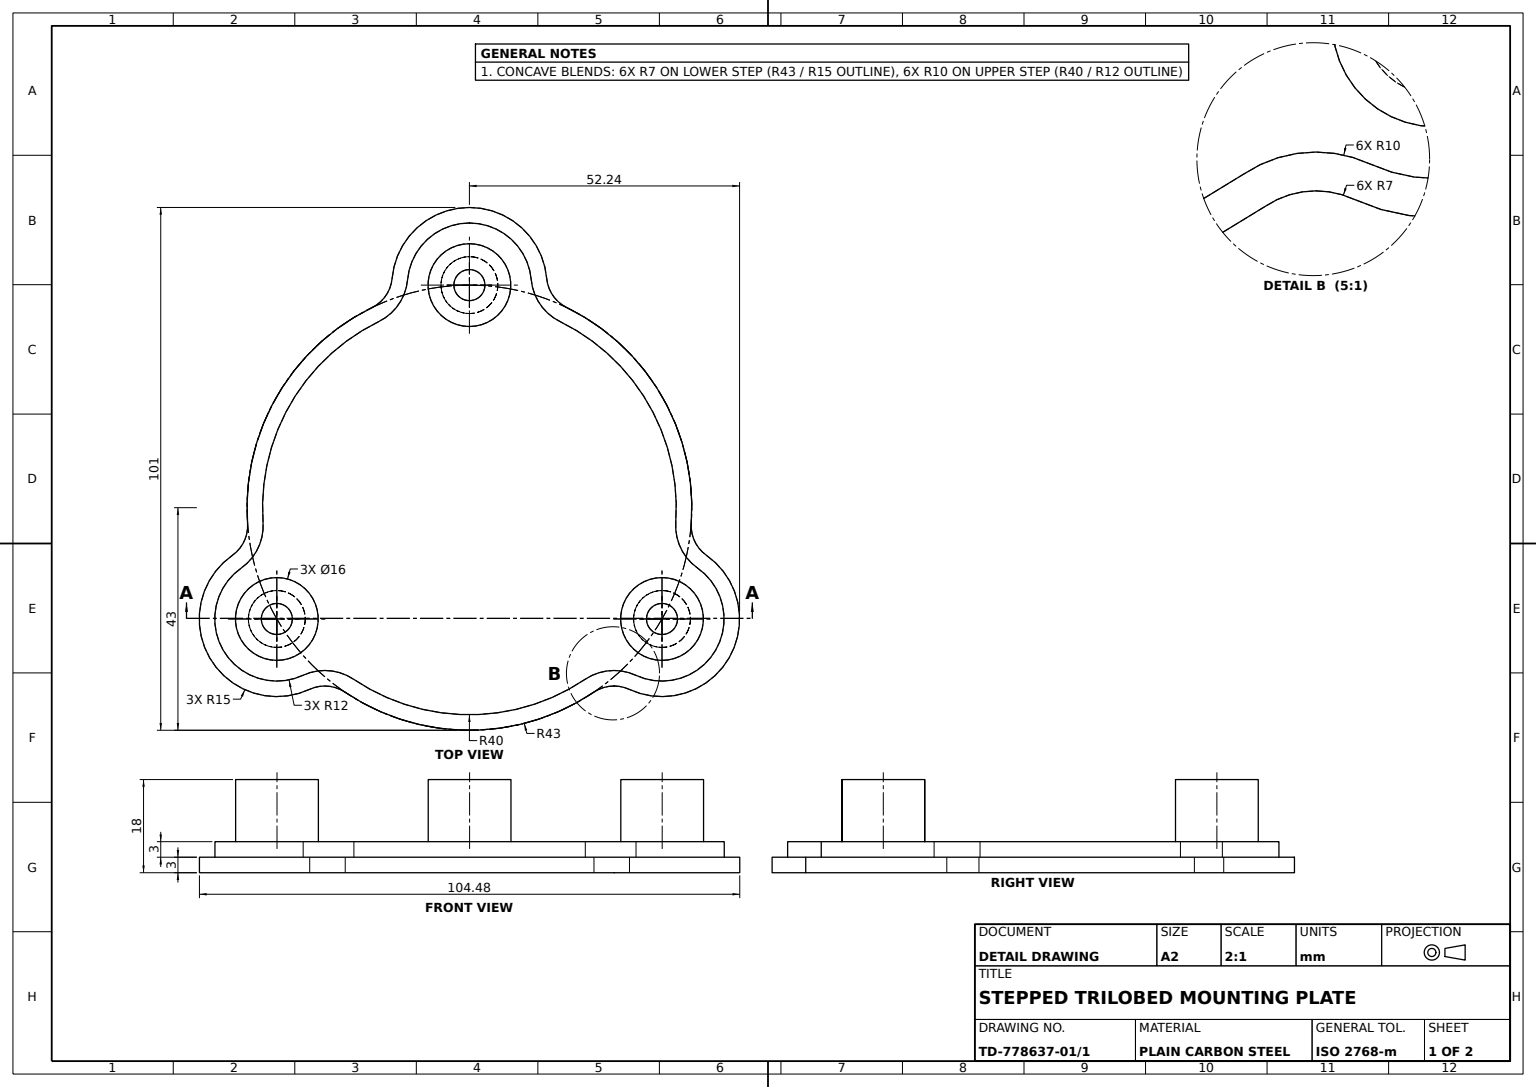
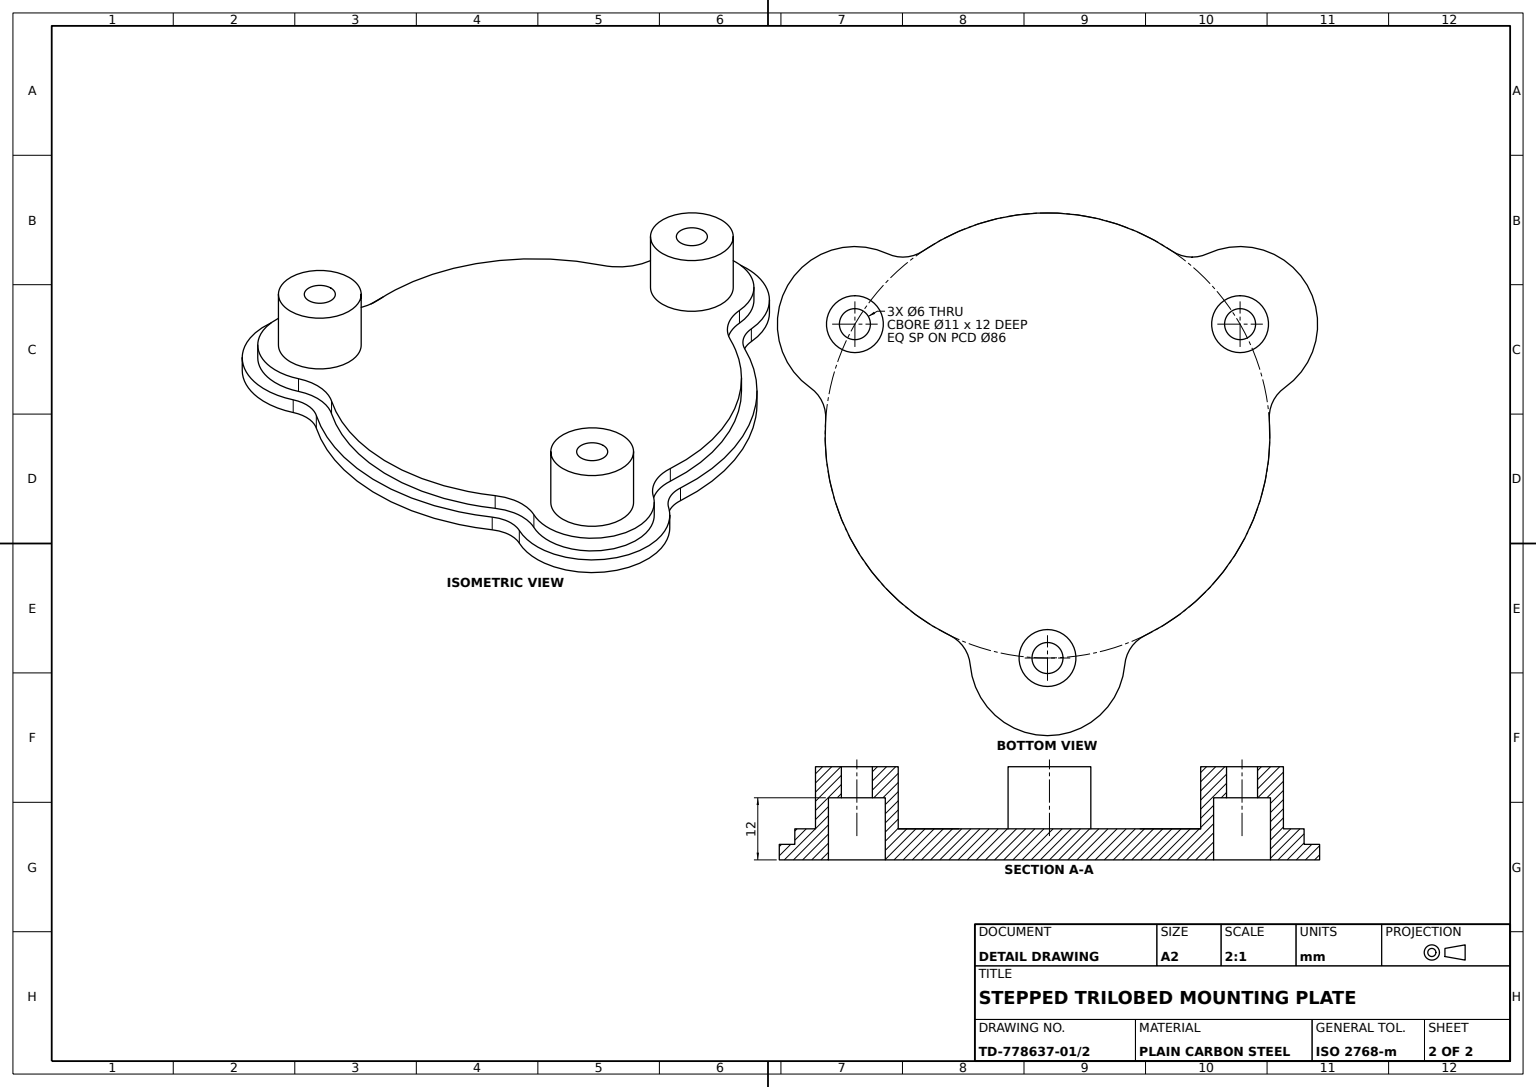
solid
v1 (27.963727,3,34.449125)
v2 (30.91498,3,35.101676)
e1 v1 v2 CIRCLE(AX(P(27.963727,3,41.449125),D(0,-1,0),D(0,0,1)),7)
v3 (27.963727,0,34.449125)
e2 v1 v3 LINE
v4 (30.91498,0,35.101676)
e3 v3 v4 CIRCLE(AX(P(27.963727,0,41.449125),D(0,-1,0),D(0,0,1)),7)
e4 v2 v4 LINE
face CYL(AX(P(27.963727,3,41.449125),D(0,-1,0),D(0,0,-1)),7) rev [-e1 e2 e3 -e4]
v5 (-37.239092,12,27)
v6 (-37.239092,12,16)
e5 v5 v6 CIRCLE(AX(P(-37.239092,12,21.5),D(0,-1,0),D(0,0,-1)),5.5)
v7 (-37.239092,0,27)
e6 v5 v7 LINE
v8 (-37.239092,0,16)
e7 v7 v8 CIRCLE(AX(P(-37.239092,0,21.5),D(0,-1,0),D(0,0,-1)),5.5)
e8 v6 v8 LINE
face CYL(AX(P(-37.239092,12,21.5),D(0,-1,0),D(0,0,-1)),5.5) rev [-e5 e6 e7 -e8]
v9 (-37.239092,18,18.5)
v10 (-37.239092,12,18.5)
e9 v9 v10 LINE
v11 (-37.239092,12,24.5)
e10 v10 v11 CIRCLE(AX(P(-37.239092,12,21.5),D(0,-1,0),D(0,0,-1)),3)
v12 (-37.239092,18,24.5)
e11 v12 v11 LINE
e12 v12 v9 CIRCLE(AX(P(-37.239092,18,21.5),D(0,1,0),D(0,0,1)),3)
face CYL(AX(P(-37.239092,22,21.5),D(0,-1,0),D(0,0,-1)),3) rev [e9 e10 -e11 e12]
v13 (-17.531306,3,-35.953488)
v14 (-39.902287,3,2.794188)
e13 v13 v14 CIRCLE(AX(P(0,3,0),D(0,1,0),D(0,0,1)),40)
v15 (-39.902287,6,2.794188)
e14 v15 v14 LINE
v16 (-17.531306,6,-35.953488)
e15 v16 v15 CIRCLE(AX(P(0,6,0),D(0,1,0),D(0,0,1)),40)
e16 v16 v13 LINE
face CYL(AX(P(0,6,0),D(0,-1,0),D(0,0,-1)),40) [e13 -e14 -e15 e16]
v17 (-44.132965,6,11.677856)
v18 (-44.132965,3,11.677856)
e17 v17 v18 LINE
v19 (-32.179802,3,32.381341)
e18 v18 v19 CIRCLE(AX(P(-37.239092,3,21.5),D(0,1,0),D(0,0,1)),12)
v20 (-32.179802,6,32.381341)
e19 v20 v19 LINE
e20 v17 v20 CIRCLE(AX(P(-37.239092,6,21.5),D(0,1,0),D(0,0,1)),12)
face CYL(AX(P(-37.239092,6,21.5),D(0,-1,0),D(0,0,-1)),12) [e17 e18 -e19 -e20]
v21 (-30.91498,0,35.101676)
v22 (-27.963727,0,34.449125)
e21 v21 v22 CIRCLE(AX(P(-27.963727,0,41.449125),D(0,-1,0),D(0,0,-1)),7)
v23 (-27.963727,3,34.449125)
e22 v23 v22 LINE
v24 (-30.91498,3,35.101676)
e23 v24 v23 CIRCLE(AX(P(-27.963727,3,41.449125),D(0,-1,0),D(0,0,-1)),7)
e24 v24 v21 LINE
face CYL(AX(P(-27.963727,3,41.449125),D(0,-1,0),D(0,0,-1)),7) rev [e21 -e22 -e23 e24]
v25 (-37.239092,6,29.5)
v26 (-37.239092,18,29.5)
e25 v25 v26 LINE
v27 (-37.239092,18,13.5)
e26 v27 v26 CIRCLE(AX(P(-37.239092,18,21.5),D(0,1,0),D(0,0,1)),8)
v28 (-37.239092,6,13.5)
e27 v28 v27 LINE
e28 v28 v25 CIRCLE(AX(P(-37.239092,6,21.5),D(0,1,0),D(0,0,1)),8)
face CYL(AX(P(-37.239092,0,21.5),D(0,1,0),D(0,0,1)),8) [e25 -e26 -e27 e28]
v29 (-27.963727,3,31.449125)
e29 v19 v29 CIRCLE(AX(P(-27.963727,3,41.449125),D(0,-1,0),D(0,0,1)),10)
v30 (-27.963727,6,31.449125)
e30 v30 v29 LINE
e31 v20 v30 CIRCLE(AX(P(-27.963727,6,41.449125),D(0,-1,0),D(0,0,1)),10)
face CYL(AX(P(-27.963727,6,41.449125),D(0,-1,0),D(0,0,-1)),10) rev [e19 e29 -e30 -e31]
e32 v26 v27 CIRCLE(AX(P(-37.239092,18,21.5),D(0,1,0),D(0,0,1)),8)
e33 v9 v12 CIRCLE(AX(P(-37.239092,18,21.5),D(0,1,0),D(0,0,1)),3)
face PLANE(AX(P(-37.239092,18,21.5),D(0,1,0),D(0,0,1))) [e26 e32] [-e33 -e12]
e34 v25 v28 CIRCLE(AX(P(-37.239092,6,21.5),D(0,1,0),D(0,0,1)),8)
face CYL(AX(P(-37.239092,0,21.5),D(0,1,0),D(0,0,1)),8) [-e32 -e25 e34 e27]
v31 (14.941454,3,-44.323996)
v32 (14.941454,0,-44.323996)
e35 v31 v32 LINE
v33 (0,0,-58)
e36 v32 v33 CIRCLE(AX(P(0,0,-43),D(0,1,0),D(0,0,1)),15)
v34 (0,3,-58)
e37 v34 v33 LINE
e38 v31 v34 CIRCLE(AX(P(0,3,-43),D(0,1,0),D(0,0,1)),15)
face CYL(AX(P(0,3,-43),D(0,-1,0),D(0,0,-1)),15) [e35 e36 -e37 -e38]
v35 (37.239092,18,18.5)
v36 (37.239092,18,24.5)
e39 v35 v36 CIRCLE(AX(P(37.239092,18,21.5),D(0,1,0),D(0,0,1)),3)
e40 v36 v35 CIRCLE(AX(P(37.239092,18,21.5),D(0,1,0),D(0,0,1)),3)
v37 (37.239092,18,13.5)
v38 (37.239092,18,29.5)
e41 v37 v38 CIRCLE(AX(P(37.239092,18,21.5),D(0,1,0),D(0,0,1)),8)
e42 v38 v37 CIRCLE(AX(P(37.239092,18,21.5),D(0,1,0),D(0,0,1)),8)
face PLANE(AX(P(37.239092,18,21.5),D(0,1,0),D(0,0,1))) [-e39 -e40] [e41 e42]
v39 (18.846153,3,-38.65)
v40 (18.846153,0,-38.65)
e43 v39 v40 LINE
e44 v40 v32 CIRCLE(AX(P(21.914132,0,-44.94186),D(0,-1,0),D(0,0,1)),7)
e45 v39 v31 CIRCLE(AX(P(21.914132,3,-44.94186),D(0,-1,0),D(0,0,1)),7)
face CYL(AX(P(21.914132,3,-44.94186),D(0,-1,0),D(0,0,-1)),7) rev [e43 e44 -e35 -e45]
v41 (24.048805,3,35.646248)
v42 (24.048805,0,35.646248)
e46 v41 v42 LINE
v43 (-24.048805,3,35.646248)
e47 v43 v41 CIRCLE(AX(P(0,3,0),D(0,1,0),D(0,0,1)),43)
v44 (-24.048805,0,35.646248)
e48 v43 v44 LINE
e49 v44 v42 CIRCLE(AX(P(0,0,0),D(0,1,0),D(0,0,1)),43)
face CYL(AX(P(0,3,0),D(0,-1,0),D(0,0,-1)),43) [-e46 -e47 e48 e49]
v45 (27.963727,6,31.449125)
v46 (27.963727,3,31.449125)
e50 v45 v46 LINE
v47 (32.179802,3,32.381341)
e51 v46 v47 CIRCLE(AX(P(27.963727,3,41.449125),D(0,-1,0),D(0,0,1)),10)
v48 (32.179802,6,32.381341)
e52 v48 v47 LINE
e53 v45 v48 CIRCLE(AX(P(27.963727,6,41.449125),D(0,-1,0),D(0,0,1)),10)
face CYL(AX(P(27.963727,6,41.449125),D(0,-1,0),D(0,0,-1)),10) rev [e50 e51 -e52 -e53]
v49 (37.239092,12,16)
v50 (37.239092,0,16)
e54 v49 v50 LINE
v51 (37.239092,12,27)
e55 v51 v49 CIRCLE(AX(P(37.239092,12,21.5),D(0,-1,0),D(0,0,-1)),5.5)
v52 (37.239092,0,27)
e56 v51 v52 LINE
e57 v52 v50 CIRCLE(AX(P(37.239092,0,21.5),D(0,-1,0),D(0,0,-1)),5.5)
face CYL(AX(P(37.239092,12,21.5),D(0,-1,0),D(0,0,-1)),5.5) rev [-e54 -e55 e56 e57]
v53 (45.856433,3,9.22232)
v54 (45.856433,0,9.22232)
e58 v53 v54 LINE
v55 (42.894959,0,3.003752)
e59 v54 v55 CIRCLE(AX(P(49.877859,0,3.492735),D(0,-1,0),D(0,0,-1)),7)
v56 (42.894959,3,3.003752)
e60 v56 v55 LINE
e61 v53 v56 CIRCLE(AX(P(49.877859,3,3.492735),D(0,-1,0),D(0,0,-1)),7)
face CYL(AX(P(49.877859,3,3.492735),D(0,-1,0),D(0,0,-1)),7) rev [e58 e59 -e60 -e61]
v57 (0,12,-40)
v58 (0,12,-46)
e62 v57 v58 CIRCLE(AX(P(0,12,-43),D(0,-1,0),D(0,0,-1)),3)
e63 v58 v57 CIRCLE(AX(P(0,12,-43),D(0,-1,0),D(0,0,-1)),3)
v59 (0,12,-48.5)
v60 (0,12,-37.5)
e64 v59 v60 CIRCLE(AX(P(0,12,-43),D(0,-1,0),D(0,0,-1)),5.5)
e65 v60 v59 CIRCLE(AX(P(0,12,-43),D(0,-1,0),D(0,0,-1)),5.5)
face PLANE(AX(P(0,12,-43),D(0,-1,0),D(0,0,-1))) [-e62 -e63] [e64 e65]
v61 (22.370982,3,33.1593)
e66 v61 v46 CIRCLE(AX(P(27.963727,3,41.449125),D(0,-1,0),D(0,0,1)),10)
v62 (22.370982,6,33.1593)
e67 v62 v45 CIRCLE(AX(P(27.963727,6,41.449125),D(0,-1,0),D(0,0,1)),10)
e68 v62 v61 LINE
face CYL(AX(P(27.963727,6,41.449125),D(0,-1,0),D(0,0,-1)),10) rev [e66 -e50 -e67 e68]
v63 (37.239092,12,18.5)
v64 (37.239092,12,24.5)
e69 v63 v64 CIRCLE(AX(P(37.239092,12,21.5),D(0,-1,0),D(0,0,-1)),3)
e70 v64 v63 CIRCLE(AX(P(37.239092,12,21.5),D(0,-1,0),D(0,0,-1)),3)
e71 v49 v51 CIRCLE(AX(P(37.239092,12,21.5),D(0,-1,0),D(0,0,-1)),5.5)
face PLANE(AX(P(37.239092,12,21.5),D(0,-1,0),D(0,0,-1))) [-e69 -e70] [e55 e71]
e72 v50 v52 CIRCLE(AX(P(37.239092,0,21.5),D(0,-1,0),D(0,0,-1)),5.5)
face CYL(AX(P(37.239092,12,21.5),D(0,-1,0),D(0,0,-1)),5.5) rev [e72 -e56 -e71 e54]
v65 (0,3,-55)
v66 (-11.953163,3,-44.059197)
e73 v65 v66 CIRCLE(AX(P(0,3,-43),D(0,1,0),D(0,0,1)),12)
v67 (-11.953163,6,-44.059197)
e74 v67 v66 LINE
v68 (0,6,-55)
e75 v68 v67 CIRCLE(AX(P(0,6,-43),D(0,1,0),D(0,0,1)),12)
e76 v68 v65 LINE
face CYL(AX(P(0,6,-43),D(0,-1,0),D(0,0,-1)),12) [e73 -e74 -e75 e76]
e77 v36 v64 LINE
e78 v35 v63 LINE
face CYL(AX(P(37.239092,22,21.5),D(0,-1,0),D(0,0,-1)),3) rev [e69 -e77 e40 e78]
e79 v41 v1 CIRCLE(AX(P(27.963727,3,41.449125),D(0,-1,0),D(0,0,1)),7)
e80 v42 v3 CIRCLE(AX(P(27.963727,0,41.449125),D(0,-1,0),D(0,0,1)),7)
face CYL(AX(P(27.963727,3,41.449125),D(0,-1,0),D(0,0,-1)),7) rev [-e79 e46 e80 -e2]
v69 (37.239092,6,29.5)
e81 v69 v38 LINE
v70 (37.239092,6,13.5)
e82 v69 v70 CIRCLE(AX(P(37.239092,6,21.5),D(0,1,0),D(0,0,1)),8)
e83 v70 v37 LINE
face CYL(AX(P(37.239092,0,21.5),D(0,1,0),D(0,0,1)),8) [-e42 -e81 e82 e83]
e84 v14 v18 CIRCLE(AX(P(-49.877859,3,3.492735),D(0,-1,0),D(0,0,1)),10)
e85 v15 v17 CIRCLE(AX(P(-49.877859,6,3.492735),D(0,-1,0),D(0,0,1)),10)
face CYL(AX(P(-49.877859,6,3.492735),D(0,-1,0),D(0,0,-1)),10) rev [e84 -e17 -e85 e14]
e86 v6 v5 CIRCLE(AX(P(-37.239092,12,21.5),D(0,-1,0),D(0,0,-1)),5.5)
e87 v11 v10 CIRCLE(AX(P(-37.239092,12,21.5),D(0,-1,0),D(0,0,-1)),3)
face PLANE(AX(P(-37.239092,12,21.5),D(0,-1,0),D(0,0,-1))) [e5 e86] [-e10 -e87]
v71 (0,18,-51)
v72 (0,18,-35)
e88 v71 v72 CIRCLE(AX(P(0,18,-43),D(0,1,0),D(0,0,1)),8)
v73 (0,6,-51)
e89 v73 v71 LINE
v74 (0,6,-35)
e90 v73 v74 CIRCLE(AX(P(0,6,-43),D(0,1,0),D(0,0,1)),8)
e91 v74 v72 LINE
face CYL(AX(P(0,0,-43),D(0,1,0),D(0,0,1)),8) [-e88 -e89 e90 e91]
face CYL(AX(P(-37.239092,22,21.5),D(0,-1,0),D(0,0,-1)),3) rev [e33 e11 e87 -e9]
v75 (44.132965,6,11.677856)
v76 (39.902287,6,2.794188)
e92 v75 v76 CIRCLE(AX(P(49.877859,6,3.492735),D(0,-1,0),D(0,0,1)),10)
v77 (44.132965,3,11.677856)
e93 v75 v77 LINE
v78 (39.902287,3,2.794188)
e94 v77 v78 CIRCLE(AX(P(49.877859,3,3.492735),D(0,-1,0),D(0,0,1)),10)
e95 v76 v78 LINE
face CYL(AX(P(49.877859,6,3.492735),D(0,-1,0),D(0,0,-1)),10) rev [-e92 e93 e94 -e95]
v79 (17.531306,6,-35.953488)
e96 v76 v79 CIRCLE(AX(P(0,6,0),D(0,1,0),D(0,0,1)),40)
v80 (17.531306,3,-35.953488)
e97 v78 v80 CIRCLE(AX(P(0,3,0),D(0,1,0),D(0,0,1)),40)
e98 v79 v80 LINE
face CYL(AX(P(0,6,0),D(0,-1,0),D(0,0,-1)),40) [-e96 e95 e97 -e98]
v81 (-42.894959,0,3.003752)
v82 (-45.856433,0,9.22232)
e99 v81 v82 CIRCLE(AX(P(-49.877859,0,3.492735),D(0,-1,0),D(0,0,1)),7)
v83 (-45.856433,3,9.22232)
e100 v83 v82 LINE
v84 (-42.894959,3,3.003752)
e101 v84 v83 CIRCLE(AX(P(-49.877859,3,3.492735),D(0,-1,0),D(0,0,1)),7)
e102 v84 v81 LINE
face CYL(AX(P(-49.877859,3,3.492735),D(0,-1,0),D(0,0,-1)),7) rev [e99 -e100 -e101 e102]
v85 (0,0,-37.5)
e103 v60 v85 LINE
v86 (0,0,-48.5)
e104 v85 v86 CIRCLE(AX(P(0,0,-43),D(0,-1,0),D(0,0,-1)),5.5)
e105 v59 v86 LINE
face CYL(AX(P(0,12,-43),D(0,-1,0),D(0,0,-1)),5.5) rev [-e65 e103 e104 -e105]
v87 (-22.370982,6,33.1593)
e106 v30 v87 CIRCLE(AX(P(-27.963727,6,41.449125),D(0,-1,0),D(0,0,1)),10)
v88 (-22.370982,3,33.1593)
e107 v29 v88 CIRCLE(AX(P(-27.963727,3,41.449125),D(0,-1,0),D(0,0,1)),10)
e108 v87 v88 LINE
face CYL(AX(P(-27.963727,6,41.449125),D(0,-1,0),D(0,0,-1)),10) rev [-e106 e30 e107 -e108]
e109 v8 v7 CIRCLE(AX(P(-37.239092,0,21.5),D(0,-1,0),D(0,0,-1)),5.5)
face CYL(AX(P(-37.239092,12,21.5),D(0,-1,0),D(0,0,-1)),5.5) rev [e8 e109 -e6 -e86]
v89 (11.953163,3,-44.059197)
e110 v89 v65 CIRCLE(AX(P(0,3,-43),D(0,1,0),D(0,0,1)),12)
e111 v80 v89 CIRCLE(AX(P(21.914132,3,-44.94186),D(0,-1,0),D(0,0,1)),10)
e112 v47 v77 CIRCLE(AX(P(37.239092,3,21.5),D(0,1,0),D(0,0,1)),12)
e113 v88 v61 CIRCLE(AX(P(0,3,0),D(0,1,0),D(0,0,1)),40)
e114 v66 v13 CIRCLE(AX(P(-21.914132,3,-44.94186),D(0,-1,0),D(0,0,1)),10)
e115 v56 v39 CIRCLE(AX(P(0,3,0),D(0,1,0),D(0,0,1)),43)
v90 (-14.941454,3,-44.323996)
e116 v34 v90 CIRCLE(AX(P(0,3,-43),D(0,1,0),D(0,0,1)),15)
v91 (-18.846153,3,-38.65)
e117 v90 v91 CIRCLE(AX(P(-21.914132,3,-44.94186),D(0,-1,0),D(0,0,-1)),7)
e118 v91 v84 CIRCLE(AX(P(0,3,0),D(0,1,0),D(0,0,1)),43)
e119 v83 v24 CIRCLE(AX(P(-37.239092,3,21.5),D(0,1,0),D(0,0,1)),15)
e120 v23 v43 CIRCLE(AX(P(-27.963727,3,41.449125),D(0,-1,0),D(0,0,-1)),7)
e121 v2 v53 CIRCLE(AX(P(37.239092,3,21.5),D(0,1,0),D(0,0,1)),15)
face PLANE(AX(P(24.938929,3,1.746368),D(0,-1,0),D(0,0,-1))) rev [-e73 -e110 -e111 -e97 -e94 -e112 -e51 -e66 -e113 -e107 -e29 -e18 -e84 -e13 -e114] [e61 e115 e45 e38 e116 e117 e118 e101 e119 e23 e120 e47 e79 e1 e121]
v92 (0,18,-46)
e122 v92 v58 LINE
v93 (0,18,-40)
e123 v92 v93 CIRCLE(AX(P(0,18,-43),D(0,1,0),D(0,0,1)),3)
e124 v93 v57 LINE
face CYL(AX(P(0,22,-43),D(0,-1,0),D(0,0,-1)),3) rev [-e122 e123 e124 e62]
e125 v82 v21 CIRCLE(AX(P(-37.239092,0,21.5),D(0,1,0),D(0,0,1)),15)
face CYL(AX(P(-37.239092,3,21.5),D(0,-1,0),D(0,0,-1)),15) [-e24 -e119 e100 e125]
e126 v22 v44 CIRCLE(AX(P(-27.963727,0,41.449125),D(0,-1,0),D(0,0,-1)),7)
face CYL(AX(P(-27.963727,3,41.449125),D(0,-1,0),D(0,0,-1)),7) rev [e22 e126 -e48 -e120]
v94 (-14.941454,0,-44.323996)
e127 v33 v94 CIRCLE(AX(P(0,0,-43),D(0,1,0),D(0,0,1)),15)
e128 v90 v94 LINE
face CYL(AX(P(0,3,-43),D(0,-1,0),D(0,0,-1)),15) [e37 e127 -e128 -e116]
v95 (-18.846153,0,-38.65)
e129 v91 v95 LINE
e130 v95 v81 CIRCLE(AX(P(0,0,0),D(0,1,0),D(0,0,1)),43)
face CYL(AX(P(0,3,0),D(0,-1,0),D(0,0,-1)),43) [-e118 e129 e130 -e102]
e131 v4 v54 CIRCLE(AX(P(37.239092,0,21.5),D(0,1,0),D(0,0,1)),15)
face CYL(AX(P(37.239092,3,21.5),D(0,-1,0),D(0,0,-1)),15) [e131 -e58 -e121 e4]
e132 v86 v85 CIRCLE(AX(P(0,0,-43),D(0,-1,0),D(0,0,-1)),5.5)
face CYL(AX(P(0,12,-43),D(0,-1,0),D(0,0,-1)),5.5) rev [-e64 e105 e132 -e103]
v96 (11.953163,6,-44.059197)
e133 v79 v96 CIRCLE(AX(P(21.914132,6,-44.94186),D(0,-1,0),D(0,0,1)),10)
e134 v96 v68 CIRCLE(AX(P(0,6,-43),D(0,1,0),D(0,0,1)),12)
e135 v67 v16 CIRCLE(AX(P(-21.914132,6,-44.94186),D(0,-1,0),D(0,0,1)),10)
e136 v87 v62 CIRCLE(AX(P(0,6,0),D(0,1,0),D(0,0,1)),40)
e137 v48 v75 CIRCLE(AX(P(37.239092,6,21.5),D(0,1,0),D(0,0,1)),12)
e138 v70 v69 CIRCLE(AX(P(37.239092,6,21.5),D(0,1,0),D(0,0,1)),8)
e139 v74 v73 CIRCLE(AX(P(0,6,-43),D(0,1,0),D(0,0,1)),8)
face PLANE(AX(P(10.957066,6,-22.47093),D(0,1,0),D(0,0,1))) [e92 e96 e133 e134 e75 e135 e15 e85 e20 e31 e106 e136 e67 e53 e137] [-e28 -e34] [-e138 -e82] [-e139 -e90]
face CYL(AX(P(-21.914132,6,-44.94186),D(0,-1,0),D(0,0,-1)),10) rev [-e135 e74 e114 -e16]
e140 v96 v89 LINE
face CYL(AX(P(0,6,-43),D(0,-1,0),D(0,0,-1)),12) [-e76 -e134 e140 e110]
e141 v94 v95 CIRCLE(AX(P(-21.914132,0,-44.94186),D(0,-1,0),D(0,0,-1)),7)
e142 v55 v40 CIRCLE(AX(P(0,0,0),D(0,1,0),D(0,0,1)),43)
face PLANE(AX(P(24.938929,0,1.746368),D(0,-1,0),D(0,0,-1))) [-e104 -e132] [-e80 -e49 -e126 -e21 -e125 -e99 -e130 -e141 -e127 -e36 -e44 -e142 -e59 -e131 -e3] [-e7 -e109] [-e57 -e72]
face CYL(AX(P(37.239092,0,21.5),D(0,1,0),D(0,0,1)),8) [e81 -e41 -e83 e138]
face CYL(AX(P(37.239092,6,21.5),D(0,-1,0),D(0,0,-1)),12) [e112 -e93 -e137 e52]
face CYL(AX(P(21.914132,6,-44.94186),D(0,-1,0),D(0,0,-1)),10) rev [-e133 e98 e111 -e140]
e143 v72 v71 CIRCLE(AX(P(0,18,-43),D(0,1,0),D(0,0,1)),8)
face CYL(AX(P(0,0,-43),D(0,1,0),D(0,0,1)),8) [e139 e89 -e143 -e91]
e144 v93 v92 CIRCLE(AX(P(0,18,-43),D(0,1,0),D(0,0,1)),3)
face CYL(AX(P(0,22,-43),D(0,-1,0),D(0,0,-1)),3) rev [e144 e122 e63 -e124]
face PLANE(AX(P(0,18,-43),D(0,1,0),D(0,0,1))) [e143 e88] [-e123 -e144]
face CYL(AX(P(0,3,0),D(0,-1,0),D(0,0,-1)),43) [e142 -e43 -e115 e60]
face CYL(AX(P(37.239092,22,21.5),D(0,-1,0),D(0,0,-1)),3) rev [e39 e77 e70 -e78]
face CYL(AX(P(0,6,0),D(0,-1,0),D(0,0,-1)),40) [-e136 e108 e113 -e68]
face CYL(AX(P(-21.914132,3,-44.94186),D(0,-1,0),D(0,0,-1)),7) rev [-e129 -e117 e128 e141]
